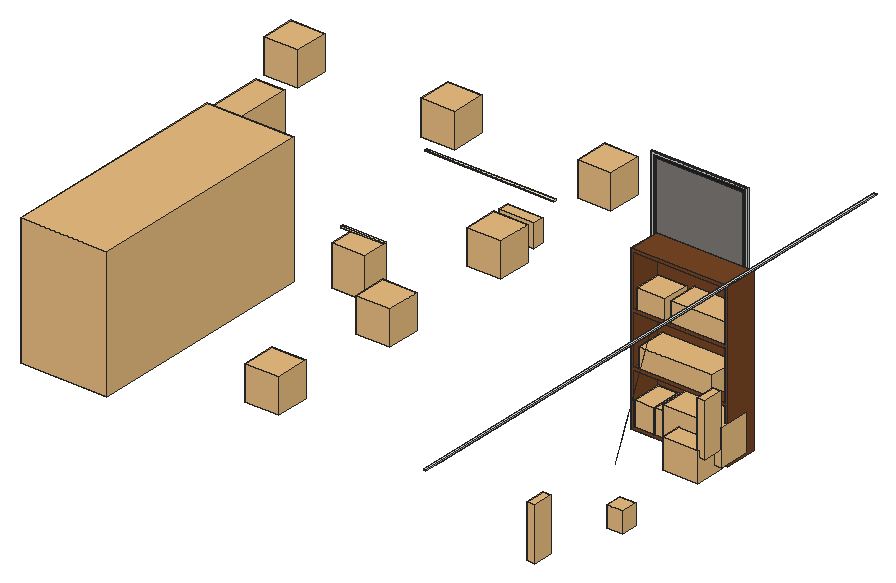
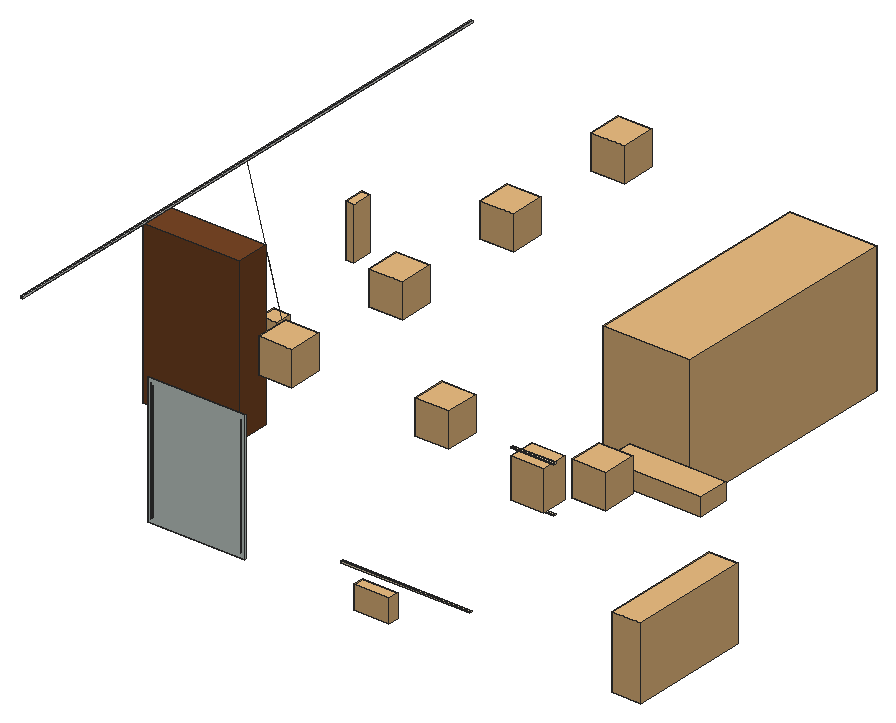
# SketchUp Ruby script. Lengths in inches.
U = 1.inch
M = Sketchup.active_model
def pt(a) = Geom::Point3d.new(a.map { |v| v * U })
def face(e, loops, mat)
  f = e.add_face(loops[0].map { |a| pt(a) })
  loops[1..].each { |l| e.add_face(l.map { |a| pt(a) }).erase! }
  f.material = f.back_material = mat if mat
  f
end
# faces: each face lists its corners as indices into pts; further lists are holes
def faces(e, pts, list, mat = nil) = list.each { |f| face(e, (f[0].is_a?(Array) ? f : [f]).map { |l| l.map { |i| pts[i] } }, mat) }
# xy, xz, yz: faces in a plane at the given z, y or x. An outline is a flat list of corners, or four numbers for a rectangle; further outlines are holes
def ring(l) = l.size == 4 ? [[l[0], l[1]], [l[2], l[1]], [l[2], l[3]], [l[0], l[3]]] : l.each_slice(2).to_a
def flat(e, list, mat, &to3) = list.each { |f| face(e, (f[0].is_a?(Array) ? f : [f]).map { |l| ring(l).map { |u, v| to3.(u, v) } }, mat) }
def xy(e, z, list, mat = nil) = flat(e, list, mat) { |x, y| [x, y, z] }
def xz(e, y, list, mat = nil) = flat(e, list, mat) { |x, z| [x, y, z] }
def yz(e, x, list, mat = nil) = flat(e, list, mat) { |y, z| [x, y, z] }
def lines(e, pts, list) = list.each { |a, b| e.add_line(pt(pts[a]), pt(pts[b])) }
# prism: a flat outline (further loops are holes) pulled along v
def prism(e, loops, v, mat = nil)
  f = face(e, loops, mat); d = Geom::Vector3d.new(v.map { |x| x * U })
  f.pushpull(f.normal.samedirection?(d) ? d.length : -d.length)
end
def box(e, o, s, mat = nil) = prism(e, [[o, [o[0] + s[0], o[1], o[2]], [o[0] + s[0], o[1] + s[1], o[2]], [o[0], o[1] + s[1], o[2]]]], [0, 0, s[2]], mat)
def at(x, y, z, deg = 0) = Geom::Transformation.translation(pt([x, y, z])) * Geom::Transformation.rotation(ORIGIN, Z_AXIS, deg.degrees)
def axes(o, x, y, z) = Geom::Transformation.new([*x, 0, *y, 0, *z, 0, *pt(o).to_a, 1])
def part(name) = M.definitions.add(name)
# library, detail: a bought-in or finely detailed component or shape, given as its bounding box
def library(name, o, s) = part(name).tap { |d| box(d.entities, o, s) }
def detail(e, o, s) = box(e.add_group.entities, o, s)
def put(e, d, t, mat = nil) = e.add_instance(d, t).tap { |i| i.material = mat if mat }
def group(e, t, mat = nil) = e.add_group.tap { |g| g.transformation = t; g.material = mat if mat }.entities
root = M.entities
M.materials.add("1467 AP 9475 Shining Blue").color = [208, 218, 214]
M.materials.add("Shelves Light").color = [249, 232, 196]
M.materials.add("Steel_ Copper_ Metal_ Aluminium").color = [30, 30, 30]
M.materials.add("[Color A01]").color = [127, 123, 119]
M.materials.add("[Wood Veneer 01]").color = [87, 43, 40]
M.materials.add("[Wood Veneer 01]1").color = [120, 70, 37]
c1 = library("Untitled\#1",[35.54,-0.34,0],[6.02,6,7.73])
c2 = library("Bathroom accessories \#1",[0,0,0],[11.95,10.24,10.01])
c3 = library("Group\#36",[0,0,-25.17],[10.55,45,26.91])
c4 = part("Group\#30")
box(c4.entities,[0,0,-0.5],[34,1,0.5])
c5 = part("wall art6")
g1 = group(c5.entities,at(66.77,0,0.01))
xy(g1,0,[[0,-0.79,39.37,0]],"Steel_ Copper_ Metal_ Aluminium")
xy(g1,0.79,[[0.79,-0.79,38.58,-0.39],[0.79,-0.39,38.58,0]],"Steel_ Copper_ Metal_ Aluminium")
xy(g1,58.27,[[0.79,-0.79,38.58,-0.39],[0.79,-0.39,38.58,0]],"Steel_ Copper_ Metal_ Aluminium")
xy(g1,59.06,[[0,-0.79,39.37,0]],"Steel_ Copper_ Metal_ Aluminium")
xz(g1,-0.79,[[[0,0,39.37,59.06],[0.79,0.79,38.58,58.27]]],"Steel_ Copper_ Metal_ Aluminium")
xz(g1,-0.39,[[0.79,0.79,38.58,58.27]],"[Color A01]")
xz(g1,0,[[[0,0,39.37,59.06],[0.79,0.79,38.58,58.27]],[0.79,0.79,38.58,58.27]],"Steel_ Copper_ Metal_ Aluminium")
yz(g1,0,[[-0.79,0,0,59.06]],"Steel_ Copper_ Metal_ Aluminium")
yz(g1,0.79,[[-0.79,0.79,-0.39,58.27],[-0.39,0.79,0,58.27]],"Steel_ Copper_ Metal_ Aluminium")
yz(g1,38.58,[[-0.79,0.79,-0.39,58.27],[-0.39,0.79,0,58.27]],"Steel_ Copper_ Metal_ Aluminium")
yz(g1,39.37,[[-0.79,0,0,59.06]],"Steel_ Copper_ Metal_ Aluminium")
c6 = library("Group\#52",[0,-0.31,0],[12.93,3.92,8.58])
c7 = library("interior plants_leaves_small",[-1.83,-3.05,0],[40.47,20.87,24.79])
c8 = library("t3",[21.64,8.43,0],[7.57,4.96,6.27])
c9 = library("Hand Towel on Rack",[0,0,0],[3.03,7.5,19.47])
c10 = library("Bahtoorm accessories \#2",[0,1.49,0],[12.27,10,14.78])
c11 = part("Group212\#1")
p = [[0,0,0],[0,0,-31.04],[-0.08,0,-31.04],[0.5,-100,0],[-0.5,-100,0],[0.5,100,0],
  [0.5,0,0],[-0.5,100,0],[0.08,0,-31.04],[-0.5,0,0],[0,0,-50.25]]
lines(c11.entities,p,[[0,1],[1,2],[3,4],[5,6],[7,5],[1,8],[9,0],[0,6],[8,10],[4,9],[6,3],[2,10],
  [9,7]])
c12 = part("Rectangle Light")
put(c12.entities,c11,at(0,0,0))
c13 = library("Umbra+Bolo",[-7.04,-1.89,-4.93],[32.14,86.7,48.29])
c14 = library("Perspective CM",[-13.58,-5.03,0],[27.16,11.23,7.55])
c15 = library("Group\#311",[0,0,0],[36,6.43,12])
c16 = library("bathroom accessories",[-9.65,-7.51,0],[20.13,16.97,7.61])
c17 = library("skp31A6",[-6.04,-1.48,32.125],[7.16,7.43,5.2])
c18 = library("4",[-4.61,-4.61,-12.6875],[12.54,12.54,12.6875])
put(root,c1,at(188.39,93.97,46),"1467 AP 9475 Shining Blue")
put(root,c2,axes([228.39,130.5,46],[-1.1,0,0],[0,1.1,0],[0,0,1.1]),"1467 AP 9475 Shining Blue")
put(root,c3,at(9,154.5,71.5),"1467 AP 9475 Shining Blue")
g2 = group(root,at(231,141,48),"[Wood Veneer 01]1")
xy(g2,0,[[-36,0,0,6],[-36,6,0,12]])
xy(g2,1,[[-35,0,-1,11]])
xy(g2,19.83,[[-35,0,-1,9],[-35,10,-1,11]])
xy(g2,20.33,[[-35,9,-1,10]])
xy(g2,20.83,[[-35,0,-1,11]])
xy(g2,39.17,[[-35,0,-1,9],[-35,10,-1,11]])
xy(g2,39.67,[[-35,9,-1,10]])
xy(g2,40.17,[[-35,0,-1,11]])
xy(g2,59,[[-35,0,-1,9],[-35,10,-1,11]])
xy(g2,59.5,[[-35,9,-1,10]])
xy(g2,60,[[-36,0,0,12]])
xz(g2,0,[[[-36,0,0,60],[-35,40.17,-1,59],[-35,1,-1,19.83],[-35,20.83,-1,39.17]]])
xz(g2,9,[[-35,19.83,-1,20.33],[-35,39.17,-1,39.67],[-35,59,-1,59.5]])
xz(g2,10,[[-35,19.83,-1,20.33],[-35,39.17,-1,39.67],[-35,59,-1,59.5]])
xz(g2,11,[[-35,1,-1,19.83],[-35,20.83,-1,39.17],[-35,40.17,-1,59]])
xz(g2,12,[[-36,0,0,60]])
yz(g2,-36,[[0,0,12,60]])
yz(g2,-35,[[0,1,11,1,11,19.83,10,19.83,10,20.33,9,20.33,9,19.83,0,19.83],[0,20.83,11,20.83,11,39.17,10,39.17,10,39.67,9,39.67,9,39.17,0,39.17],[0,40.17,11,40.17,11,59,10,59,10,59.5,9,59.5,9,59,0,59]])
yz(g2,-1,[[0,1,0,19.83,9,19.83,9,20.33,10,20.33,10,19.83,11,19.83,11,1],[0,20.83,0,39.17,9,39.17,9,39.67,10,39.67,10,39.17,11,39.17,11,20.83],[0,40.17,0,59,9,59,9,59.5,10,59.5,10,59,11,59,11,40.17]])
yz(g2,0,[[0,0,12,60]])
put(g2,c4,at(-35,9,59.5),"Shelves Light")
put(g2,c4,at(-35,9,39.67),"Shelves Light")
put(g2,c4,at(-35,9,20.33),"Shelves Light")
g3 = group(root,at(150,207,48),"1467 AP 9475 Shining Blue")
xy(g3,0,[[0,-0.5,36,0]])
xy(g3,1,[[1,-0.5,35,-0.25]])
xy(g3,47,[[1,-0.5,35,-0.25]])
xy(g3,48,[[0,-0.5,36,0]])
xz(g3,-0.5,[[[0,0,36,48],[1,1,35,47]]])
xz(g3,-0.25,[[1,1,35,47]])
xz(g3,0,[[0,0,36,48]])
yz(g3,0,[[-0.5,0,0,48]])
yz(g3,1,[[-0.5,1,-0.25,47]])
yz(g3,35,[[-0.5,1,-0.25,47]])
yz(g3,36,[[-0.5,0,0,48]])
put(g3,c5,axes([-56.66,-0.25,0.99],[0.8636,0,0],[0,0.3175,0],[0,0,0.77893]))
put(root,c6,at(93.6,207,48))
put(root,c7,axes([210.4,139.53,48.95],[0.54,0,0],[0,0.54,0],[0,0,0.54]))
put(root,c8,axes([184.26,183.36,49],[0,-1.45,0],[1.45,0,0],[0,0,1.45]))
put(root,c8,axes([191.76,183.36,58.09],[0,-1.45,0],[1.45,0,0],[0,0,-1.45]))
put(root,c9,at(227.6,52.06,54.6875),"1467 AP 9475 Shining Blue")
put(root,c9,at(227.6,130.92,54.6875),"1467 AP 9475 Shining Blue")
g4 = group(root,at(85,144,58.5),"Shelves Light")
box(g4,[0,0,-0.5],[16,1,0.5])
put(root,c10,at(87.32,135.26,59),"1467 AP 9475 Shining Blue")
g5 = group(root,at(230,1,108.01))
box(g5,[0,0,0],[1,209,0.5])
put(g5,c12,axes([0.5,104.5,-0.01],[-0.96593,0,0.25882],[0,1,0],[0.25882,0,0.96593]))
g6 = group(root,at(62.5,211,63.5),"Shelves Light")
box(g6,[0,0,-0.5],[48,1,0.5])
put(root,c13,at(75.95,122.6,69.5625,180),"1467 AP 9475 Shining Blue")
put(root,c14,at(211.66,146.03,68.83),"1467 AP 9475 Shining Blue")
put(root,c15,axes([36,138,72],[1,0,0],[0,0,1],[0,-1,0]),"[Wood Veneer 01]")
g7 = group(root,at(85,144,75.5),"Shelves Light")
box(g7,[0,0,-0.5],[16,1,0.5])
put(root,c16,axes([219.52,145.87,88.17],[1,0,0],[0,0.64822,0],[0,0,1]))
put(root,c17,axes([199.23,142.59,42.87],[0,-1.41,0],[1.41,0,0],[0,0,1.41]))
put(root,c18,at(38.34,176.84,108))
put(root,c18,at(96.59,176.84,108))
put(root,c18,at(154.84,176.84,108))
put(root,c18,at(154.84,125.34,108))
put(root,c18,at(154.84,73.84,108))
put(root,c18,at(154.84,22.34,108))
